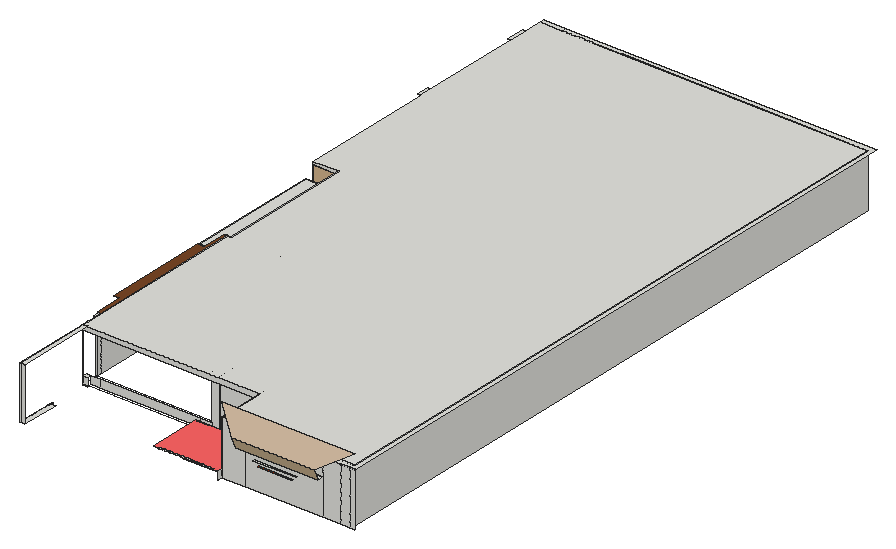
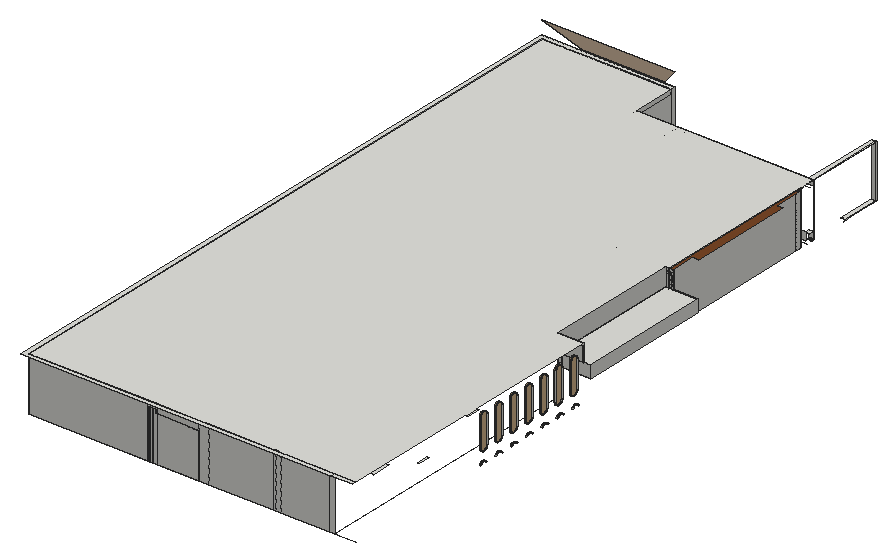
# SketchUp Ruby script. Lengths in inches.
U = 1.inch
M = Sketchup.active_model
def pt(a) = Geom::Point3d.new(a.map { |v| v * U })
def face(e, loops, mat)
  f = e.add_face(loops[0].map { |a| pt(a) })
  loops[1..].each { |l| e.add_face(l.map { |a| pt(a) }).erase! }
  f.material = f.back_material = mat if mat
  f
end
# faces: each face lists its corners as indices into pts; further lists are holes
def faces(e, pts, list, mat = nil) = list.each { |f| face(e, (f[0].is_a?(Array) ? f : [f]).map { |l| l.map { |i| pts[i] } }, mat) }
# xy, xz, yz: faces in a plane at the given z, y or x. An outline is a flat list of corners, or four numbers for a rectangle; further outlines are holes
def ring(l) = l.size == 4 ? [[l[0], l[1]], [l[2], l[1]], [l[2], l[3]], [l[0], l[3]]] : l.each_slice(2).to_a
def flat(e, list, mat, &to3) = list.each { |f| face(e, (f[0].is_a?(Array) ? f : [f]).map { |l| ring(l).map { |u, v| to3.(u, v) } }, mat) }
def xy(e, z, list, mat = nil) = flat(e, list, mat) { |x, y| [x, y, z] }
def xz(e, y, list, mat = nil) = flat(e, list, mat) { |x, z| [x, y, z] }
def yz(e, x, list, mat = nil) = flat(e, list, mat) { |y, z| [x, y, z] }
def lines(e, pts, list) = list.each { |a, b| e.add_line(pt(pts[a]), pt(pts[b])) }
# prism: a flat outline (further loops are holes) pulled along v
def prism(e, loops, v, mat = nil)
  f = face(e, loops, mat); d = Geom::Vector3d.new(v.map { |x| x * U })
  f.pushpull(f.normal.samedirection?(d) ? d.length : -d.length)
end
def box(e, o, s, mat = nil) = prism(e, [[o, [o[0] + s[0], o[1], o[2]], [o[0] + s[0], o[1] + s[1], o[2]], [o[0], o[1] + s[1], o[2]]]], [0, 0, s[2]], mat)
def at(x, y, z, deg = 0) = Geom::Transformation.translation(pt([x, y, z])) * Geom::Transformation.rotation(ORIGIN, Z_AXIS, deg.degrees)
def axes(o, x, y, z) = Geom::Transformation.new([*x, 0, *y, 0, *z, 0, *pt(o).to_a, 1])
def part(name) = M.definitions.add(name)
# library, detail: a bought-in or finely detailed component or shape, given as its bounding box
def library(name, o, s) = part(name).tap { |d| box(d.entities, o, s) }
def detail(e, o, s) = box(e.add_group.entities, o, s)
def put(e, d, t, mat = nil) = e.add_instance(d, t).tap { |i| i.material = mat if mat }
def group(e, t, mat = nil) = e.add_group.tap { |g| g.transformation = t; g.material = mat if mat }.entities
root = M.entities
M.materials.add("[0035_Tan]").color = [210, 180, 140]
M.materials.add("[Color A03]").color = [255, 101, 101]
M.materials.add("[Color B07]").color = [153, 38, 0]
M.materials.add("[Formica Beige]").color = [211, 187, 149]
M.materials.add("[Formica Laminate Light]").color = [213, 189, 164]
M.materials.add("[Wood Veneer 01]").color = [120, 70, 37]
xy(root,358.375,[[436.61,51.9375,436.79,59.45],[450.77,68.37,450.77,68.42,454.96,68.41,454.96,68.37],[454.96,68.37,454.96,68.41,482.19,68.37],[482.19,68.37,454.96,68.41,454.96,1311.7,686.08,1311.7,686.08,68.37],[454.96,68.41,450.77,68.42,454.96,68.42],
  [355.71,68.42,436.61,151.375],[436.61,68.42,436.61,151.375,445.61,151.375,445.61,68.43,445.79,68.43,450.77,68.42],[450.77,68.42,445.79,68.43,445.79,151.375,450.77,151.375],[450.77,68.42,454.96,151.375],[445.61,68.43,445.79,151.375],
  [94.33,151.375,102.83,154.81],[336.9375,151.375,436.61,154.81],[436.61,151.375,436.61,154.81,355.71,154.81,355.71,160.375,445.61,160.375,445.61,151.375],[445.61,151.375,445.79,160.375],[445.79,151.375,450.77,160.375],
  [450.77,151.375,454.96,160.375],[94.33,154.81,102.83,155],[336.9375,154.81,355.71,160.375],[336.9375,160.375,355.71,167.06],[355.71,160.375,445.61,1311.7],
  [445.61,160.375,450.77,1311.7],[450.77,160.375,454.96,1311.7],[336.9375,167.06,355.71,186.31],[336.9375,186.31,355.71,1311.7]])
xy(root,360,[[93.83,0,94.14,68.42],[94.14,0,94.33,68.42],[94.33,0,102.83,73.57],[93.83,68.42,94.14,73.57],[94.14,68.42,94.33,73.57]])
xy(root,373.8125,[[323.875,48.9375,331.3125,51.9375],[334.4375,48.9375,341.875,51.9375],[345,48.9375,352.4375,51.9375],[355.5625,48.9375,363,51.9375],[366.125,48.9375,373.5625,51.9375],
  [376.6875,48.9375,384.125,51.9375],[387.25,48.9375,394.6875,51.9375],[397.8125,48.9375,405.25,51.9375],[408.375,48.9375,415.8125,51.9375],[418.9375,48.9375,426.375,51.9375],
  [445.61,68.43,445.79,160.375],[94.14,151.375,102.83,160.375]])
xy(root,373.8125,[[313.3125,48.9375,320.75,48.9375,320.75,51.9375,429.5,51.9375,429.5,48.9375,436.61,48.9375,436.61,151.375,313.3125,151.375]],"[Color A03]")
xy(root,394.5,[[97.83,570.62,100.83,675.43]])
xy(root,403.875,[[93.83,499.93,208.04,508.43]])
xy(root,405.25,[[87.77,501.15,87.77,501.9,38.21,501.9,38.21,760.27,93.83,760.27,93.83,761.77,100.83,761.77,100.83,501.15]])
xy(root,411.49,[[517.45,44.37,582.95,47.37]],"[Color B07]")
xy(root,419.48,[[509.46,44.37,590.93,47.37]])
xy(root,427.93,[[473.83,47.37,632.12,59.37]])
xy(root,429.125,[[87.77,501.15,100.83,501.15,100.83,761.77,93.83,761.77,93.83,760.27,38.21,760.27,38.21,501.9,87.77,501.9],[38.21,501.27,87.77,501.9],[52.02,760.27,93.83,761.77]])
xy(root,430.9375,[[48.64,1140.89,51.64,1161.64]])
xy(root,445.625,[[355.71,160.375,440.45,1311.7]])
xy(root,453.125,[[436.61,68.42,445.61,68.43],[445.61,68.42,450.77,68.42,445.79,68.43,445.61,68.43],[450.77,68.42,450.77,160.375,445.61,160.375,445.61,68.43,445.79,68.43],[450.77,68.42,454.96,160.375],[436.61,68.43,440.45,151.375],
  [336.9375,151.375,355.71,154.81],[355.71,151.375,436.61,154.81],[436.61,151.375,440.45,160.375],[440.45,151.375,445.61,160.375],[336.9375,154.81,355.71,160.375],
  [355.71,154.81,436.61,160.375],[440.45,160.375,445.61,1311.7],[445.61,160.375,450.77,1311.7],[450.77,160.375,454.96,1311.7]])
xy(root,457.125,[[52.02,760.27,93.83,761.77]])
xy(root,463.1875,[[93.83,0,94.14,151.375],[94.14,0,94.33,151.375],[94.33,0,102.83,151.375],[482.18,59.37,695.08,59.37,695.08,1320.7,93.83,1320.7,93.83,1311.7,686.08,1311.7,686.08,68.37,450.77,68.37,450.77,68.42,436.61,68.42,436.61,59.45,436.98,59.45,437.36,59.44],[482.19,68.37,686.08,68.37,686.08,1311.7,51.64,1311.7,51.64,1047.49,48.64,1047.49,48.64,1022.51,51.64,1022.51,51.64,761.77,100.83,761.77,100.83,501.15,93.83,501.15,93.83,488.08,94.14,488.08,94.14,151.375,436.61,151.375,436.61,68.43,445.61,68.43,450.77,68.42,454.96,68.42,454.96,68.41],
  [450.77,68.37,454.96,68.37,454.96,68.41,450.77,68.42],[454.96,68.37,482.19,68.37,454.96,68.41],[454.96,68.41,454.96,68.42,450.77,68.42],[436.61,68.42,445.61,68.43],[445.61,68.42,450.77,68.42,445.61,68.43],
  [93.83,151.375,94.14,154.81],[93.83,154.81,94.14,160.375],[93.83,160.375,94.14,167.06],[93.83,167.06,94.14,186.31],[90.83,182.28,93.83,194.66],
  [93.83,186.31,94.14,488.08],[45.64,1022.51,48.64,1047.49],[45.64,1240.86,51.64,1277.54],[51.64,1311.7,93.83,1320.7]])
xz(root,0,[[93.83,360,94.14,463.1875],[94.14,360,94.33,463.1875],[94.33,360,102.83,463.1875]])
xz(root,59.37,[[482.18,358.375,632.12,427.93],[632.12,358.375,666.86,463.1875],[666.86,358.375,684.83,463.1875],[684.83,358.375,693.83,463.1875],[693.83,358.375,695.08,463.1875],
  [482.18,427.93,632.12,463.1875]])
xz(root,59.45,[[436.61,358.375,436.79,463.1875],[436.79,358.375,436.98,463.1875]])
xz(root,68.37,[[450.77,358.375,454.96,463.1875],[454.96,358.375,482.19,463.1875],[482.19,358.375,632.12,463.1875],[632.12,358.375,666.86,463.1875],[666.86,358.375,684.83,463.1875],
  [684.83,358.375,686.08,463.1875]])
xz(root,68.42,[[436.61,358.375,450.77,453.125],[450.77,358.375,454.96,453.125],[436.61,453.125,445.61,463.1875],[445.61,453.125,450.77,463.1875],[450.77,453.125,454.96,463.1875]])
xz(root,68.43,[[445.61,358.375,445.79,373.8125],[436.61,373.8125,445.61,453.125],[445.61,373.8125,445.79,453.125],[436.61,453.125,440.45,463.1875],[440.45,453.125,445.61,463.1875]])
xz(root,73.57,[[93.83,359.47,94.14,360],[94.14,359.47,94.33,360],[94.33,359.47,102.83,360]])
xz(root,151.375,[[93.83,358.375,94.14,360],[94.14,358.375,94.33,360],[94.33,358.375,102.83,360],[313.3125,358.375,336.9375,373.8125],[436.61,358.375,445.61,453.125],
  [93.83,360,94.14,373.8125],[94.14,360,94.33,373.8125],[94.33,360,102.83,373.8125],[93.83,373.8125,94.33,453.125],[93.83,453.125,94.33,463.1875],
  [94.33,453.125,436.61,463.1875]])
xz(root,154.81,[[355.71,358.375,436.61,453.125]])
xz(root,160.375,[[102.83,358.375,120.24,373.8125],[120.24,358.375,313.3125,373.8125],[313.3125,358.375,336.9375,373.8125],[336.9375,358.375,445.61,358.375,445.61,453.125,440.45,453.125,440.45,445.625,355.71,445.625,355.71,453.125,336.9375,453.125],[445.61,358.375,445.79,373.8125],
  [355.71,445.625,436.61,453.125],[436.61,445.625,440.45,453.125]])
xz(root,501.15,[[93.83,358.375,100.83,405.25],[87.77,405.25,87.83,413.4375],[87.83,405.25,87.83,413.4375,93.32,413.4375,93.24,405.25],[93.24,405.25,93.32,405.25,93.32,413.4375],[93.32,405.25,93.48,413.4375],
  [93.48,405.25,93.77,413.4375],[93.77,405.25,93.83,413.4375],[93.83,405.25,100.83,413.4375],[87.77,413.4375,87.83,429.125],[87.83,413.4375,87.83,429.125,93.48,429.125,93.32,413.4375],
  [93.32,413.4375,93.48,413.4375,93.48,429.125],[93.48,413.4375,93.77,429.125],[93.77,413.4375,93.83,429.125],[93.83,413.4375,100.83,429.125],[87.77,429.125,87.83,453.5625],
  [87.83,429.125,93.48,453.5625],[93.48,429.125,93.48,453.5625,93.73,453.5625],[93.48,429.125,93.77,429.125,93.77,453.5625,93.73,453.5625],[93.77,429.125,93.83,453.5625],[93.83,429.125,100.83,453.5625],
  [87.77,453.5625,87.83,457.125],[87.83,453.5625,87.83,457.125,93.77,457.125,93.73,453.5625],[93.73,453.5625,93.77,453.5625,93.77,457.125],[93.77,453.5625,93.83,457.125],[93.83,453.5625,100.83,457.125],
  [87.77,457.125,87.83,463.1875,87.83,457.125],[87.83,457.125,87.83,463.1875,93.83,463.1875,93.77,457.125],[93.77,457.125,93.83,463.1875,93.83,457.125],[93.83,457.125,100.83,463.1875],[87.83,463.1875,87.83,463.25,93.83,463.1875]])
xz(root,501.9,[[38.21,405.25,87.77,429.125]])
xz(root,760.27,[[38.21,405.25,93.83,429.125]])
xz(root,760.27,[[52.02,429.125,93.83,457.125]],"[0035_Tan]")
xz(root,761.77,[[93.83,405.25,100.83,413.4375],[93.83,413.4375,100.83,429.125],[51.64,429.125,52.02,457.125],[93.83,429.125,100.83,429.125,100.83,463.1875,51.64,463.1875,51.64,457.125,93.83,457.125],[52.02,429.125,93.83,457.125]])
xz(root,761.77,[[93.83,358.375,100.83,405.25]],"[0035_Tan]")
xz(root,776.11,[[51.64,388.28,54.64,443.41]])
xz(root,791.55,[[51.64,388.28,54.64,443.41]])
xz(root,812.49,[[51.64,388.28,55.14,443.41]])
xz(root,827.93,[[51.64,388.28,55.14,443.41]])
xz(root,848.86,[[51.64,388.28,54.64,443.41]])
xz(root,864.3,[[51.64,388.28,54.64,443.41]])
xz(root,885.24,[[51.64,388.28,54.64,443.41]])
xz(root,900.68,[[51.64,388.28,54.64,443.41]])
xz(root,921.61,[[51.64,388.28,54.64,443.41]])
xz(root,937.05,[[51.64,388.28,54.64,443.41]])
xz(root,957.99,[[51.64,388.28,54.64,443.41]])
xz(root,973.43,[[51.64,388.28,54.64,443.41]])
xz(root,994.36,[[51.64,388.28,54.64,443.41]])
xz(root,1009.8,[[51.64,388.28,54.64,443.41]])
xz(root,1311.7,[[93.83,358.375,102.83,463.1875],[102.83,358.375,197.39,463.1875],[197.39,358.375,208.04,463.1875],[208.04,358.375,210.36,463.1875],[210.36,358.375,336.9375,463.1875],
  [336.9375,358.375,355.71,463.1875],[355.71,358.375,436.7,445.625],[436.7,358.375,436.7,445.625,440.45,445.625,440.45,453.125,445.61,453.125,445.61,358.375],[445.61,358.375,450.77,453.125],[450.77,358.375,454.96,453.125],
  [454.96,358.375,686.08,463.1875],[355.71,445.625,436.7,463.1875],[436.7,445.625,440.45,463.1875],[440.45,453.125,445.61,463.1875],[445.61,453.125,454.96,463.1875]])
yz(root,38.21,[[501.9,405.25,760.27,429.125]])
yz(root,52.02,[[760.27,429.125,761.77,457.125]])
yz(root,54.64,[[783.83,380.5625,781.83,380.83,779.97,381.6,778.375,382.82,777.15,384.42,776.375,386.28,776.11,388.28,776.11,443.41,776.72,445.06,777.67,446.53,778.93,447.77,780.42,448.69,782.08,449.27,783.83,449.46,785.58,449.27,787.24,448.69,788.74,447.77,789.99,446.53,790.95,445.06,791.55,443.41,791.55,388.28,791.29,386.28,790.52,384.42,789.29,382.82,787.69,381.6,785.83,380.83],[856.58,380.5625,854.58,380.83,852.72,381.6,851.125,382.82,849.9,384.42,849.125,386.28,848.86,388.28,848.86,443.41,849.47,445.06,850.42,446.53,851.68,447.77,853.17,448.69,854.83,449.27,856.58,449.46,858.33,449.27,859.99,448.69,861.49,447.77,862.74,446.53,863.7,445.06,864.3,443.41,864.3,388.28,864.04,386.28,863.27,384.42,862.04,382.82,860.44,381.6,858.58,380.83],[892.96,380.5625,890.96,380.83,889.1,381.6,887.5,382.82,886.27,384.42,885.5,386.28,885.24,388.28,885.24,443.41,885.84,445.06,886.8,446.53,888.05,447.77,889.55,448.69,891.21,449.27,892.96,449.46,894.7,449.27,896.37,448.69,897.86,447.77,899.12,446.53,900.07,445.06,900.68,443.41,900.68,388.28,900.41,386.28,899.64,384.42,898.41,382.82,896.82,381.6,894.95,380.83],[929.33,380.5625,927.33,380.83,925.47,381.6,923.875,382.82,922.65,384.42,921.875,386.28,921.61,388.28,921.61,443.41,922.22,445.06,923.17,446.53,924.43,447.77,925.92,448.69,927.58,449.27,929.33,449.46,931.08,449.27,932.74,448.69,934.24,447.77,935.49,446.53,936.45,445.06,937.05,443.41,937.05,388.28,936.79,386.28,936.02,384.42,934.79,382.82,933.19,381.6,931.33,380.83],[965.71,380.5625,963.71,380.83,961.85,381.6,960.25,382.82,959.02,384.42,958.25,386.28,957.99,388.28,957.99,443.41,958.59,445.06,959.55,446.53,960.8,447.77,962.3,448.69,963.96,449.27,965.71,449.46,967.45,449.27,969.12,448.69,970.61,447.77,971.87,446.53,972.82,445.06,973.43,443.41,973.43,388.28,973.16,386.28,972.39,384.42,971.16,382.82,969.57,381.6,967.7,380.83],
  [1002.08,380.5625,1000.08,380.83,998.22,381.6,996.625,382.82,995.4,384.42,994.625,386.28,994.36,388.28,994.36,443.41,994.97,445.06,995.92,446.53,997.18,447.77,998.67,448.69,1000.33,449.27,1002.08,449.46,1003.83,449.27,1005.49,448.69,1006.99,447.77,1008.24,446.53,1009.2,445.06,1009.8,443.41,1009.8,388.28,1009.54,386.28,1008.77,384.42,1007.54,382.82,1005.94,381.6,1004.08,380.83]],"[0035_Tan]")
yz(root,55.14,[[820.21,380.5625,818.21,380.83,816.35,381.6,814.75,382.82,813.52,384.42,812.75,386.28,812.49,388.28,812.49,443.41,813.09,445.06,814.05,446.53,815.3,447.77,816.8,448.69,818.46,449.27,820.21,449.46,821.95,449.27,823.62,448.69,825.11,447.77,826.37,446.53,827.32,445.06,827.93,443.41,827.93,388.28,827.66,386.28,826.89,384.42,825.66,382.82,824.07,381.6,822.2,380.83]],"[0035_Tan]")
yz(root,87.77,[[501.15,405.25,501.27,413.4375],[501.27,405.25,501.9,413.4375],[501.15,413.4375,501.27,429.125],[501.27,413.4375,501.9,429.125],[501.15,429.125,501.27,453.5625],
  [501.27,429.125,501.9,453.5625],[501.15,453.5625,501.27,457.125],[501.27,453.5625,501.9,457.125]])
yz(root,93.83,[[68.42,358.375,68.42,360,73.57,360,73.57,359.47,78.72,358.375],[182.28,358.375,186.31,360],[186.31,358.375,194.66,463.1875],[194.66,358.375,488.08,463.1875],[488.08,358.375,488.08,463.1875,500.32,463.1875,500.32,403.875,499.93,403.875,499.93,358.375],
  [499.93,358.375,500.32,403.875],[500.32,358.375,501.15,403.875],[182.28,360,186.31,463.1875],[500.32,403.875,501.15,463.1875],[760.27,405.25,761.77,413.4375],
  [760.27,413.4375,761.77,429.125],[760.27,429.125,761.77,453.5625],[760.27,453.5625,761.77,457.125]])
yz(root,100.83,[[501.15,405.25,761.77,413.4375],[501.15,413.4375,761.77,429.125],[501.15,429.125,761.77,463.1875]])
yz(root,355.71,[[154.81,358.375,167.06,358.375,167.06,445.625,160.375,445.625,160.375,453.125,154.81,453.125],[167.06,358.375,186.31,445.625],[186.31,358.375,1311.7,445.625]])
yz(root,436.61,[[48.9375,358.375,59.45,373.8125],[59.45,358.375,68.42,373.8125],[68.42,358.375,151.375,373.8125],[151.375,358.375,154.81,453.125],[59.45,373.8125,68.42,463.1875],
  [68.42,373.8125,68.43,453.125],[68.43,373.8125,151.375,453.125],[68.42,453.125,68.43,463.1875],[68.43,453.125,151.375,463.1875]])
yz(root,440.45,[[160.375,445.625,1311.7,453.125]])
yz(root,445.61,[[68.43,358.375,151.375,373.8125],[151.375,358.375,160.375,373.8125],[160.375,358.375,1311.7,453.125],[68.43,373.8125,151.375,453.125],[68.42,453.125,68.43,463.1875]])
yz(root,445.79,[[68.43,358.375,160.375,373.8125]])
yz(root,450.77,[[68.37,358.375,68.42,463.1875],[68.42,358.375,1311.7,453.125]])
yz(root,454.96,[[68.37,358.375,68.42,463.1875],[68.42,358.375,1311.7,453.125]])
yz(root,686.08,[[68.37,358.375,1311.7,463.1875]])
p = [[436.98,59.45,358.375],[437.36,59.44,358.375],[437.36,59.44,463.1875],[436.98,59.45,463.1875],[482.18,59.37,358.375],[482.18,59.37,427.93],
  [482.18,59.37,463.1875],[445.61,68.43,453.125],[445.79,68.43,453.125],[450.77,68.42,453.125],[450.77,68.42,358.375],[445.79,68.43,358.375],
  [445.61,68.43,358.375],[445.61,68.43,373.8125],[445.79,68.43,373.8125],[454.96,68.41,358.375],[450.77,68.42,463.1875],[454.96,68.41,463.1875],
  [482.19,68.37,463.1875],[482.19,68.37,358.375],[93.83,73.57,359.47],[93.83,78.72,358.375],[94.14,78.72,358.375],[94.14,73.57,359.47],
  [94.33,78.72,358.375],[94.33,73.57,359.47],[51.64,771.84,358.74],[51.64,772.8,360.22],[54.64,772.8,360.22],[54.64,771.84,358.74],
  [51.64,785.12,360.22],[51.64,786.07,358.74],[54.64,786.07,358.74],[54.64,785.12,360.22],[51.64,809.03,358.74],[51.64,809.98,360.22],
  [55.14,809.98,360.22],[55.14,809.03,358.74],[51.64,822.3,360.22],[51.64,823.26,358.74],[55.14,823.26,358.74],[55.14,822.3,360.22],
  [51.64,846.22,358.74],[51.64,847.17,360.22],[54.64,847.17,360.22],[54.64,846.22,358.74],[51.64,859.49,360.22],[51.64,860.45,358.74],
  [54.64,860.45,358.74],[54.64,859.49,360.22],[51.64,883.41,358.74],[51.64,884.36,360.22],[54.64,884.36,360.22],[54.64,883.41,358.74],
  [51.64,896.68,360.22],[51.64,897.63,358.74],[54.64,897.63,358.74],[54.64,896.68,360.22],[51.64,920.59,358.74],[51.64,921.55,360.22],
  [54.64,921.55,360.22],[54.64,920.59,358.74],[51.64,933.87,360.22],[51.64,934.82,358.74],[54.64,934.82,358.74],[54.64,933.87,360.22],
  [51.64,957.78,358.74],[51.64,958.73,360.22],[54.64,958.73,360.22],[54.64,957.78,358.74],[51.64,971.05,360.22],[51.64,972.01,358.74],
  [54.64,972.01,358.74],[54.64,971.05,360.22],[51.64,994.97,358.74],[51.64,995.92,360.22],[54.64,995.92,360.22],[54.64,994.97,358.74],
  [51.64,1008.24,360.22],[51.64,1009.2,358.74],[54.64,1009.2,358.74],[54.64,1008.24,360.22],[51.64,774.05,361.45],[54.64,774.05,361.45],
  [51.64,783.86,361.45],[54.64,783.86,361.45],[51.64,811.24,361.45],[55.14,811.24,361.45],[51.64,821.05,361.45],[55.14,821.05,361.45],
  [51.64,848.43,361.45],[54.64,848.43,361.45],[51.64,858.24,361.45],[54.64,858.24,361.45],[51.64,885.61,361.45],[54.64,885.61,361.45],
  [51.64,895.42,361.45],[54.64,895.42,361.45],[51.64,922.8,361.45],[54.64,922.8,361.45],[51.64,932.61,361.45],[54.64,932.61,361.45],
  [51.64,959.99,361.45],[54.64,959.99,361.45],[51.64,969.8,361.45],[54.64,969.8,361.45],[51.64,997.18,361.45],[54.64,997.18,361.45],
  [51.64,1006.99,361.45],[54.64,1006.99,361.45],[51.64,775.55,362.38],[54.64,775.55,362.38],[51.64,782.37,362.38],[54.64,782.37,362.38],
  [51.64,812.73,362.38],[55.14,812.73,362.38],[51.64,819.55,362.38],[55.14,819.55,362.38],[51.64,849.92,362.38],[54.64,849.92,362.38],
  [51.64,856.74,362.38],[54.64,856.74,362.38],[51.64,887.11,362.38],[54.64,887.11,362.38],[51.64,893.93,362.38],[54.64,893.93,362.38],
  [51.64,924.3,362.38],[54.64,924.3,362.38],[51.64,931.12,362.38],[54.64,931.12,362.38],[51.64,961.48,362.38],[54.64,961.48,362.38],
  [51.64,968.3,362.38],[54.64,968.3,362.38],[51.64,998.67,362.38],[54.64,998.67,362.38],[51.64,1005.49,362.38],[54.64,1005.49,362.38],
  [51.64,777.21,362.95],[54.64,777.21,362.95],[51.64,780.7,362.95],[54.64,780.7,362.95],[51.64,814.4,362.95],[55.14,814.4,362.95],
  [51.64,817.89,362.95],[55.14,817.89,362.95],[51.64,851.58,362.95],[54.64,851.58,362.95],[51.64,855.08,362.95],[54.64,855.08,362.95],
  [51.64,888.77,362.95],[54.64,888.77,362.95],[51.64,892.27,362.95],[54.64,892.27,362.95],[51.64,925.96,362.95],[54.64,925.96,362.95],
  [51.64,929.45,362.95],[54.64,929.45,362.95],[51.64,963.15,362.95],[54.64,963.15,362.95],[51.64,966.64,362.95],[54.64,966.64,362.95],
  [51.64,1000.33,362.95],[54.64,1000.33,362.95],[51.64,1003.83,362.95],[54.64,1003.83,362.95],[51.64,778.96,363.15],[54.64,778.96,363.15],
  [51.64,816.14,363.15],[55.14,816.14,363.15],[51.64,853.33,363.15],[54.64,853.33,363.15],[51.64,890.52,363.15],[54.64,890.52,363.15],
  [51.64,927.71,363.15],[54.64,927.71,363.15],[51.64,964.89,363.15],[54.64,964.89,363.15],[51.64,1002.08,363.15],[54.64,1002.08,363.15],
  [51.64,783.83,380.5625],[51.64,781.83,380.83],[54.64,781.83,380.83],[54.64,783.83,380.5625],[51.64,785.83,380.83],[54.64,785.83,380.83],
  [51.64,820.21,380.5625],[51.64,818.21,380.83],[55.14,818.21,380.83],[55.14,820.21,380.5625],[51.64,822.2,380.83],[55.14,822.2,380.83],
  [51.64,856.58,380.5625],[51.64,854.58,380.83],[54.64,854.58,380.83],[54.64,856.58,380.5625],[51.64,858.58,380.83],[54.64,858.58,380.83],
  [51.64,892.96,380.5625],[51.64,890.96,380.83],[54.64,890.96,380.83],[54.64,892.96,380.5625],[51.64,894.95,380.83],[54.64,894.95,380.83],
  [51.64,929.33,380.5625],[51.64,927.33,380.83],[54.64,927.33,380.83],[54.64,929.33,380.5625],[51.64,931.33,380.83],[54.64,931.33,380.83],
  [51.64,965.71,380.5625],[51.64,963.71,380.83],[54.64,963.71,380.83],[54.64,965.71,380.5625],[51.64,967.7,380.83],[54.64,967.7,380.83],
  [51.64,1002.08,380.5625],[51.64,1000.08,380.83],[54.64,1000.08,380.83],[54.64,1002.08,380.5625],[51.64,1004.08,380.83],[54.64,1004.08,380.83],
  [51.64,779.97,381.6],[54.64,779.97,381.6],[51.64,787.69,381.6],[54.64,787.69,381.6],[51.64,816.35,381.6],[55.14,816.35,381.6],
  [51.64,824.07,381.6],[55.14,824.07,381.6],[51.64,852.72,381.6],[54.64,852.72,381.6],[51.64,860.44,381.6],[54.64,860.44,381.6],
  [51.64,889.1,381.6],[54.64,889.1,381.6],[51.64,896.82,381.6],[54.64,896.82,381.6],[51.64,925.47,381.6],[54.64,925.47,381.6],
  [51.64,933.19,381.6],[54.64,933.19,381.6],[51.64,961.85,381.6],[54.64,961.85,381.6],[51.64,969.57,381.6],[54.64,969.57,381.6],
  [51.64,998.22,381.6],[54.64,998.22,381.6],[51.64,1005.94,381.6],[54.64,1005.94,381.6],[51.64,778.375,382.82],[54.64,778.375,382.82],
  [51.64,789.29,382.82],[54.64,789.29,382.82],[51.64,814.75,382.82],[55.14,814.75,382.82],[51.64,825.66,382.82],[55.14,825.66,382.82],
  [51.64,851.125,382.82],[54.64,851.125,382.82],[51.64,862.04,382.82],[54.64,862.04,382.82],[51.64,887.5,382.82],[54.64,887.5,382.82],
  [51.64,898.41,382.82],[54.64,898.41,382.82],[51.64,923.875,382.82],[54.64,923.875,382.82],[51.64,934.79,382.82],[54.64,934.79,382.82],
  [51.64,960.25,382.82],[54.64,960.25,382.82],[51.64,971.16,382.82],[54.64,971.16,382.82],[51.64,996.625,382.82],[54.64,996.625,382.82],
  [51.64,1007.54,382.82],[54.64,1007.54,382.82],[51.64,777.15,384.42],[54.64,777.15,384.42],[51.64,790.52,384.42],[54.64,790.52,384.42],
  [51.64,813.52,384.42],[55.14,813.52,384.42],[51.64,826.89,384.42],[55.14,826.89,384.42],[51.64,849.9,384.42],[54.64,849.9,384.42],
  [51.64,863.27,384.42],[54.64,863.27,384.42],[51.64,886.27,384.42],[54.64,886.27,384.42],[51.64,899.64,384.42],[54.64,899.64,384.42],
  [51.64,922.65,384.42],[54.64,922.65,384.42],[51.64,936.02,384.42],[54.64,936.02,384.42],[51.64,959.02,384.42],[54.64,959.02,384.42],
  [51.64,972.39,384.42],[54.64,972.39,384.42],[51.64,995.4,384.42],[54.64,995.4,384.42],[51.64,1008.77,384.42],[54.64,1008.77,384.42],
  [51.64,776.375,386.28],[54.64,776.375,386.28],[51.64,791.29,386.28],[54.64,791.29,386.28],[51.64,812.75,386.28],[55.14,812.75,386.28],
  [51.64,827.66,386.28],[55.14,827.66,386.28],[51.64,849.125,386.28],[54.64,849.125,386.28],[51.64,864.04,386.28],[54.64,864.04,386.28],
  [51.64,885.5,386.28],[54.64,885.5,386.28],[51.64,900.41,386.28],[54.64,900.41,386.28],[51.64,921.875,386.28],[54.64,921.875,386.28],
  [51.64,936.79,386.28],[54.64,936.79,386.28],[51.64,958.25,386.28],[54.64,958.25,386.28],[51.64,973.16,386.28],[54.64,973.16,386.28],
  [51.64,994.625,386.28],[54.64,994.625,386.28],[51.64,1009.54,386.28],[54.64,1009.54,386.28],[51.64,776.11,388.28],[54.64,776.11,388.28],
  [51.64,791.55,388.28],[54.64,791.55,388.28],[51.64,812.49,388.28],[55.14,812.49,388.28],[51.64,827.93,388.28],[55.14,827.93,388.28],
  [51.64,848.86,388.28],[54.64,848.86,388.28],[51.64,864.3,388.28],[54.64,864.3,388.28],[51.64,885.24,388.28],[54.64,885.24,388.28],
  [51.64,900.68,388.28],[54.64,900.68,388.28],[51.64,921.61,388.28],[54.64,921.61,388.28],[51.64,937.05,388.28],[54.64,937.05,388.28],
  [51.64,957.99,388.28],[54.64,957.99,388.28],[51.64,973.43,388.28],[54.64,973.43,388.28],[51.64,994.36,388.28],[54.64,994.36,388.28],
  [51.64,1009.8,388.28],[54.64,1009.8,388.28],[473.83,47.37,427.93],[632.12,47.37,427.93],[632.12,37.62,450.15],[473.83,37.62,450.15],
  [51.64,776.11,443.41],[51.64,776.72,445.06],[54.64,776.72,445.06],[54.64,776.11,443.41],[51.64,790.95,445.06],[51.64,791.55,443.41],
  [54.64,791.55,443.41],[54.64,790.95,445.06],[51.64,812.49,443.41],[51.64,813.09,445.06],[55.14,813.09,445.06],[55.14,812.49,443.41],
  [51.64,827.32,445.06],[51.64,827.93,443.41],[55.14,827.93,443.41],[55.14,827.32,445.06],[51.64,848.86,443.41],[51.64,849.47,445.06],
  [54.64,849.47,445.06],[54.64,848.86,443.41],[51.64,863.7,445.06],[51.64,864.3,443.41],[54.64,864.3,443.41],[54.64,863.7,445.06],
  [51.64,885.24,443.41],[51.64,885.84,445.06],[54.64,885.84,445.06],[54.64,885.24,443.41],[51.64,900.07,445.06],[51.64,900.68,443.41],
  [54.64,900.68,443.41],[54.64,900.07,445.06],[51.64,921.61,443.41],[51.64,922.22,445.06],[54.64,922.22,445.06],[54.64,921.61,443.41],
  [51.64,936.45,445.06],[51.64,937.05,443.41],[54.64,937.05,443.41],[54.64,936.45,445.06],[51.64,957.99,443.41],[51.64,958.59,445.06],
  [54.64,958.59,445.06],[54.64,957.99,443.41],[51.64,972.82,445.06],[51.64,973.43,443.41],[54.64,973.43,443.41],[54.64,972.82,445.06],
  [51.64,994.36,443.41],[51.64,994.97,445.06],[54.64,994.97,445.06],[54.64,994.36,443.41],[51.64,1009.2,445.06],[51.64,1009.8,443.41],
  [54.64,1009.8,443.41],[54.64,1009.2,445.06],[51.64,777.67,446.53],[54.64,777.67,446.53],[51.64,789.99,446.53],[54.64,789.99,446.53],
  [51.64,814.05,446.53],[55.14,814.05,446.53],[51.64,826.37,446.53],[55.14,826.37,446.53],[51.64,850.42,446.53],[54.64,850.42,446.53],
  [51.64,862.74,446.53],[54.64,862.74,446.53],[51.64,886.8,446.53],[54.64,886.8,446.53],[51.64,899.12,446.53],[54.64,899.12,446.53],
  [51.64,923.17,446.53],[54.64,923.17,446.53],[51.64,935.49,446.53],[54.64,935.49,446.53],[51.64,959.55,446.53],[54.64,959.55,446.53],
  [51.64,971.87,446.53],[54.64,971.87,446.53],[51.64,995.92,446.53],[54.64,995.92,446.53],[51.64,1008.24,446.53],[54.64,1008.24,446.53],
  [51.64,778.93,447.77],[54.64,778.93,447.77],[51.64,788.74,447.77],[54.64,788.74,447.77],[51.64,815.3,447.77],[55.14,815.3,447.77],
  [51.64,825.11,447.77],[55.14,825.11,447.77],[51.64,851.68,447.77],[54.64,851.68,447.77],[51.64,861.49,447.77],[54.64,861.49,447.77],
  [51.64,888.05,447.77],[54.64,888.05,447.77],[51.64,897.86,447.77],[54.64,897.86,447.77],[51.64,924.43,447.77],[54.64,924.43,447.77],
  [51.64,934.24,447.77],[54.64,934.24,447.77],[51.64,960.8,447.77],[54.64,960.8,447.77],[51.64,970.61,447.77],[54.64,970.61,447.77],
  [51.64,997.18,447.77],[54.64,997.18,447.77],[51.64,1006.99,447.77],[54.64,1006.99,447.77],[51.64,780.42,448.69],[54.64,780.42,448.69],
  [51.64,787.24,448.69],[54.64,787.24,448.69],[51.64,816.8,448.69],[55.14,816.8,448.69],[51.64,823.62,448.69],[55.14,823.62,448.69],
  [51.64,853.17,448.69],[54.64,853.17,448.69],[51.64,859.99,448.69],[54.64,859.99,448.69],[51.64,889.55,448.69],[54.64,889.55,448.69],
  [51.64,896.37,448.69],[54.64,896.37,448.69],[51.64,925.92,448.69],[54.64,925.92,448.69],[51.64,932.74,448.69],[54.64,932.74,448.69],
  [51.64,962.3,448.69],[54.64,962.3,448.69],[51.64,969.12,448.69],[54.64,969.12,448.69],[51.64,998.67,448.69],[54.64,998.67,448.69],
  [51.64,1005.49,448.69],[54.64,1005.49,448.69],[51.64,782.08,449.27],[54.64,782.08,449.27],[51.64,785.58,449.27],[54.64,785.58,449.27],
  [51.64,818.46,449.27],[55.14,818.46,449.27],[51.64,821.95,449.27],[55.14,821.95,449.27],[51.64,854.83,449.27],[54.64,854.83,449.27],
  [51.64,858.33,449.27],[54.64,858.33,449.27],[51.64,891.21,449.27],[54.64,891.21,449.27],[51.64,894.7,449.27],[54.64,894.7,449.27],
  [51.64,927.58,449.27],[54.64,927.58,449.27],[51.64,931.08,449.27],[54.64,931.08,449.27],[51.64,963.96,449.27],[54.64,963.96,449.27],
  [51.64,967.45,449.27],[54.64,967.45,449.27],[51.64,1000.33,449.27],[54.64,1000.33,449.27],[51.64,1003.83,449.27],[54.64,1003.83,449.27],
  [51.64,783.83,449.46],[54.64,783.83,449.46],[51.64,820.21,449.46],[55.14,820.21,449.46],[51.64,856.58,449.46],[54.64,856.58,449.46],
  [51.64,892.96,449.46],[54.64,892.96,449.46],[51.64,929.33,449.46],[54.64,929.33,449.46],[51.64,965.71,449.46],[54.64,965.71,449.46],
  [51.64,1002.08,449.46],[54.64,1002.08,449.46],[693.83,59.37,489.375],[436.7,59.37,489.375],[445.61,68.43,463.1875],[93.83,500.32,463.1875],
  [93.83,501.15,463.1875],[87.83,501.15,463.25],[87.83,452.86,463.25],[75.83,452.86,463.37],[75.83,249.3,463.37],[87.83,249.3,463.25],
  [87.83,194.66,463.25],[93.83,194.66,463.1875],[93.83,488.08,463.1875],[102.83,59.45,359.47],[102.83,73.57,359.47],[102.83,501.15,463.1875],
  [102.83,501.15,461.25],[197.39,501.15,463.1875],[197.39,501.15,461.25],[93.83,1311.7,358.375],[51.64,1311.7,358.375],[93.83,761.77,358.375],
  [336.9375,160.375,453.125],[336.9375,160.375,463.1875],[94.14,160.375,373.8125],[93.83,160.375,373.8125],[336.9375,186.31,358.375],[93.83,186.31,358.375],
  [336.9375,167.06,358.375],[93.83,167.06,358.375],[336.9375,154.81,358.375],[102.83,154.81,358.375],[93.83,160.375,453.125],[436.61,160.375,463.1875],
  [436.61,160.375,453.125],[355.71,160.375,463.1875],[355.71,160.375,453.125],[355.71,186.31,445.625],[355.71,186.31,463.1875],[355.71,167.06,445.625],
  [355.71,167.06,463.1875],[355.71,154.81,453.125],[355.71,154.81,463.1875],[102.83,759.83,461.25],[197.39,759.83,461.25],[87.83,501.15,463.1875],
  [87.83,501.9,463.1875],[94.33,154.81,358.375],[93.83,154.81,358.375]]
faces(root,p,[[0,1,2,3],[1,4,5,6,2],[7,8,9,10,11,12,13],[10,11,14,8,9],[15,10,9,16,17,18,19],[20,21,22,23],[23,22,24,25],[26,27,28,29],
  [30,31,32,33],[34,35,36,37],[38,39,40,41],[42,43,44,45],[46,47,48,49],[50,51,52,53],[54,55,56,57],[58,59,60,61],
  [62,63,64,65],[66,67,68,69],[70,71,72,73],[74,75,76,77],[78,79,80,81],[27,82,83,28],[84,30,33,85],[35,86,87,36],
  [88,38,41,89],[43,90,91,44],[92,46,49,93],[51,94,95,52],[96,54,57,97],[59,98,99,60],[100,62,65,101],[67,102,103,68],
  [104,70,73,105],[75,106,107,76],[108,78,81,109],[82,110,111,83],[112,84,85,113],[86,114,115,87],[116,88,89,117],[90,118,119,91],
  [120,92,93,121],[94,122,123,95],[124,96,97,125],[98,126,127,99],[128,100,101,129],[102,130,131,103],[132,104,105,133],[106,134,135,107],
  [136,108,109,137],[110,138,139,111],[140,112,113,141],[114,142,143,115],[144,116,117,145],[118,146,147,119],[148,120,121,149],[122,150,151,123],
  [152,124,125,153],[126,154,155,127],[156,128,129,157],[130,158,159,131],[160,132,133,161],[134,162,163,135],[164,136,137,165],[138,166,167,139],
  [166,140,141,167],[142,168,169,143],[168,144,145,169],[146,170,171,147],[170,148,149,171],[150,172,173,151],[172,152,153,173],[154,174,175,155],
  [174,156,157,175],[158,176,177,159],[176,160,161,177],[162,178,179,163],[178,164,165,179],[180,181,182,183],[184,180,183,185],[186,187,188,189],
  [190,186,189,191],[192,193,194,195],[196,192,195,197],[198,199,200,201],[202,198,201,203],[204,205,206,207],[208,204,207,209],[210,211,212,213],
  [214,210,213,215],[216,217,218,219],[220,216,219,221],[181,222,223,182],[224,184,185,225],[187,226,227,188],[228,190,191,229],[193,230,231,194],
  [232,196,197,233],[199,234,235,200],[236,202,203,237],[205,238,239,206],[240,208,209,241],[211,242,243,212],[244,214,215,245],[217,246,247,218],
  [248,220,221,249],[222,250,251,223],[252,224,225,253],[226,254,255,227],[256,228,229,257],[230,258,259,231],[260,232,233,261],[234,262,263,235],
  [264,236,237,265],[238,266,267,239],[268,240,241,269],[242,270,271,243],[272,244,245,273],[246,274,275,247],[276,248,249,277],[250,278,279,251],
  [280,252,253,281],[254,282,283,255],[284,256,257,285],[258,286,287,259],[288,260,261,289],[262,290,291,263],[292,264,265,293],[266,294,295,267],
  [296,268,269,297],[270,298,299,271],[300,272,273,301],[274,302,303,275],[304,276,277,305],[278,306,307,279],[308,280,281,309],[282,310,311,283],
  [312,284,285,313],[286,314,315,287],[316,288,289,317],[290,318,319,291],[320,292,293,321],[294,322,323,295],[324,296,297,325],[298,326,327,299],
  [328,300,301,329],[302,330,331,303],[332,304,305,333],[306,334,335,307],[336,308,309,337],[310,338,339,311],[340,312,313,341],[314,342,343,315],
  [344,316,317,345],[318,346,347,319],[348,320,321,349],[322,350,351,323],[352,324,325,353],[326,354,355,327],[356,328,329,357],[330,358,359,331],
  [360,332,333,361],[366,367,368,369],[370,371,372,373],[374,375,376,377],[378,379,380,381],[382,383,384,385],[386,387,388,389],[390,391,392,393],
  [394,395,396,397],[398,399,400,401],[402,403,404,405],[406,407,408,409],[410,411,412,413],[414,415,416,417],[418,419,420,421],[367,422,423,368],
  [424,370,373,425],[375,426,427,376],[428,378,381,429],[383,430,431,384],[432,386,389,433],[391,434,435,392],[436,394,397,437],[399,438,439,400],
  [440,402,405,441],[407,442,443,408],[444,410,413,445],[415,446,447,416],[448,418,421,449],[422,450,451,423],[452,424,425,453],[426,454,455,427],
  [456,428,429,457],[430,458,459,431],[460,432,433,461],[434,462,463,435],[464,436,437,465],[438,466,467,439],[468,440,441,469],[442,470,471,443],
  [472,444,445,473],[446,474,475,447],[476,448,449,477],[450,478,479,451],[480,452,453,481],[454,482,483,455],[484,456,457,485],[458,486,487,459],
  [488,460,461,489],[462,490,491,463],[492,464,465,493],[466,494,495,467],[496,468,469,497],[470,498,499,471],[500,472,473,501],[474,502,503,475],
  [504,476,477,505],[478,506,507,479],[508,480,481,509],[482,510,511,483],[512,484,485,513],[486,514,515,487],[516,488,489,517],[490,518,519,491],
  [520,492,493,521],[494,522,523,495],[524,496,497,525],[498,526,527,499],[528,500,501,529],[502,530,531,503],[532,504,505,533],[506,534,535,507],
  [534,508,509,535],[510,536,537,511],[536,512,513,537],[514,538,539,515],[538,516,517,539],[518,540,541,519],[540,520,521,541],[522,542,543,523],
  [542,524,525,543],[526,544,545,527],[544,528,529,545],[530,546,547,531],[546,532,533,547],[550,16,9,8,7]])
faces(root,p,[[362,363,364,365]],"[Formica Beige]")
faces(root,p,[[364,548,549,365]],"[Formica Laminate Light]")
faces(root,p,[[551,552,553,554,555,556,557,558,559,560]],"[Wood Veneer 01]")
lines(root,p,[[561,562],[563,564],[565,566],[567,568],[569,567],[570,571],[572,573],[574,575],[576,577],[578,579],[570,580],[581,582],
  [583,584],[585,586],[587,588],[589,590],[591,564],[592,566],[593,594],[595,596]])
